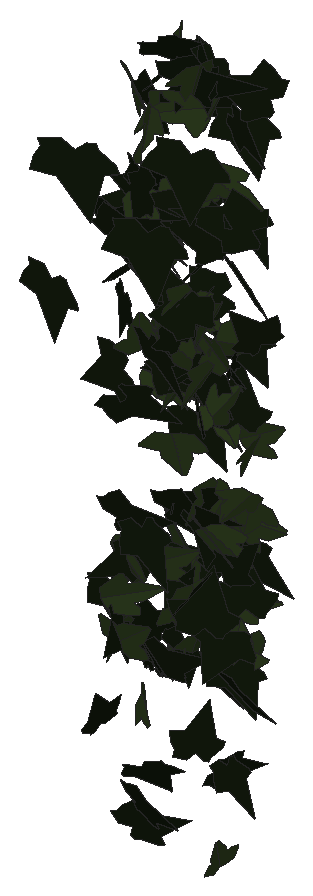
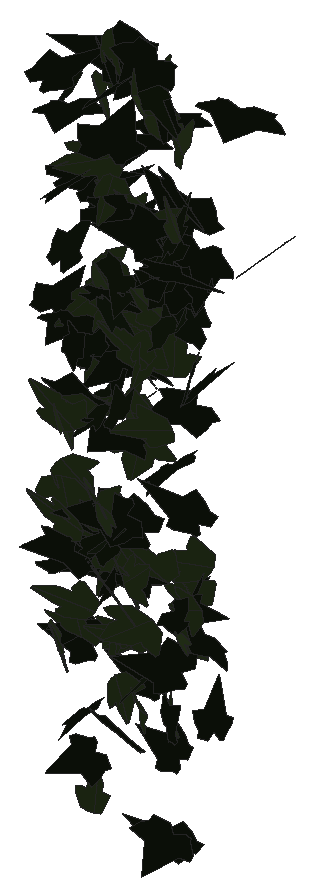
# SketchUp Ruby script. Lengths in inches.
U = 1.inch
M = Sketchup.active_model
def pt(a) = Geom::Point3d.new(a.map { |v| v * U })
def face(e, loops, mat)
  f = e.add_face(loops[0].map { |a| pt(a) })
  loops[1..].each { |l| e.add_face(l.map { |a| pt(a) }).erase! }
  f.material = f.back_material = mat if mat
  f
end
# faces: each face lists its corners as indices into pts; further lists are holes
def faces(e, pts, list, mat = nil) = list.each { |f| face(e, (f[0].is_a?(Array) ? f : [f]).map { |l| l.map { |i| pts[i] } }, mat) }
# xy, xz, yz: faces in a plane at the given z, y or x. An outline is a flat list of corners, or four numbers for a rectangle; further outlines are holes
def ring(l) = l.size == 4 ? [[l[0], l[1]], [l[2], l[1]], [l[2], l[3]], [l[0], l[3]]] : l.each_slice(2).to_a
def flat(e, list, mat, &to3) = list.each { |f| face(e, (f[0].is_a?(Array) ? f : [f]).map { |l| ring(l).map { |u, v| to3.(u, v) } }, mat) }
def xy(e, z, list, mat = nil) = flat(e, list, mat) { |x, y| [x, y, z] }
def xz(e, y, list, mat = nil) = flat(e, list, mat) { |x, z| [x, y, z] }
def yz(e, x, list, mat = nil) = flat(e, list, mat) { |y, z| [x, y, z] }
def lines(e, pts, list) = list.each { |a, b| e.add_line(pt(pts[a]), pt(pts[b])) }
# prism: a flat outline (further loops are holes) pulled along v
def prism(e, loops, v, mat = nil)
  f = face(e, loops, mat); d = Geom::Vector3d.new(v.map { |x| x * U })
  f.pushpull(f.normal.samedirection?(d) ? d.length : -d.length)
end
def box(e, o, s, mat = nil) = prism(e, [[o, [o[0] + s[0], o[1], o[2]], [o[0] + s[0], o[1] + s[1], o[2]], [o[0], o[1] + s[1], o[2]]]], [0, 0, s[2]], mat)
def at(x, y, z, deg = 0) = Geom::Transformation.translation(pt([x, y, z])) * Geom::Transformation.rotation(ORIGIN, Z_AXIS, deg.degrees)
def axes(o, x, y, z) = Geom::Transformation.new([*x, 0, *y, 0, *z, 0, *pt(o).to_a, 1])
def part(name) = M.definitions.add(name)
# library, detail: a bought-in or finely detailed component or shape, given as its bounding box
def library(name, o, s) = part(name).tap { |d| box(d.entities, o, s) }
def detail(e, o, s) = box(e.add_group.entities, o, s)
def put(e, d, t, mat = nil) = e.add_instance(d, t).tap { |i| i.material = mat if mat }
def group(e, t, mat = nil) = e.add_group.tap { |g| g.transformation = t; g.material = mat if mat }.entities
root = M.entities
M.materials.add("1026 AP 7946 SUNNY SIDE UP").color = [254, 231, 186]
M.materials.add("efeu1").color = [18, 25, 13]
M.materials.add("efeu2").color = [43, 57, 29]
c1 = part("ivyleaf_9")
p = [[1.54,2.16,1.25],[1.36,2.04,1.19],[-0.21,0.99,0.68],[-0.71,1.11,0.82],[-0.85,0.86,0.67],[-0.8,0.17,0.21],
  [-0.9,-0.01,0.1],[-0.67,-0.16,-0.02],[-0.08,-0.08,-0.05],[-0.03,-0.6,-0.4],[0.65,-0.88,-0.66],[0.83,-0.6,-0.49],
  [1.29,-0.42,-0.43],[1.8125,-0.07,-0.26],[1.21,0.44,0.15]]
faces(c1.entities,p,[[0,1,2,3,4,5,6,7,8,9,10,11,12,13,14]],"efeu1")
c2 = part("ivyleaf_10")
p = [[0,0.5,-0.03],[-0.0625,2.02,-0.43],[-0.19,2.01,-0.46],[-0.54,1.05,-0.29],[-0.52,0.625,-0.18],[-0.83,0.76,-0.28],
  [-1.16,0.64,-0.33],[-1.15,0.33,-0.24],[-0.77,-0.39,0.02],[-0.3,-0.51,0.16],[0.04,-0.48,0.23],[-0.02,2.01,-0.4375],
  [-0.06,2.01,-0.43],[0.04,-0.49,0.23],[0.67,-0.49,0.14],[1.38,0.36,-0.2],[1.375,0.51,-0.24],[0.81,0.65,-0.19],
  [0.62,0.59,-0.15],[0.6,1.09,-0.28],[0.5,1.23,-0.31]]
faces(c2.entities,p,[[0,1,2,3,4,5,6,7,8,9,10],[11,12,0,13,14,15,16,17,18,19,20]],"efeu2")
put(root,c1,axes([121.75,208.88,265.58],[-0.19201,-0.31929,-0.11255],[0.08789,0.09349,-0.35114],[0.52237,-0.1331,0.01771]),"1026 AP 7946 SUNNY SIDE UP")
put(root,c1,axes([119.59,209.1,263.89],[-0.01059,-0.33233,0.09962],[-0.00328,-0.09857,-0.34301],[0.54506,-0.00705,-0.00013]),"1026 AP 7946 SUNNY SIDE UP")
put(root,c1,axes([120.09,209.08,266.43],[-0.28859,-0.21576,-0.21786],[0.23882,0.14635,-0.29045],[0.40909,-0.23764,0.01587]),"1026 AP 7946 SUNNY SIDE UP")
put(root,c2,axes([122.375,209.58,262.97],[0.06672,-0.23881,0.21649],[0.04615,-0.20954,-0.25103],[0.49948,0.05126,-0.00572]),"1026 AP 7946 SUNNY SIDE UP")
put(root,c1,axes([121.18,209.46,259.69],[0.07711,-0.30009,-0.11327],[-0.0425,0.10522,-0.31249],[0.49982,0.05524,-0.0091]),"1026 AP 7946 SUNNY SIDE UP")
put(root,c2,axes([121.8,209.7,264.09],[0.07309,-0.17687,0.28511],[0.07156,-0.27437,-0.18944],[0.51282,0.06349,-0.0142]),"1026 AP 7946 SUNNY SIDE UP")
put(root,c2,axes([120.71,209.5,257.46],[-0.38346,-0.00104,0.19279],[0.29295,0.0277,0.25043],[-0.02781,0.30615,-0.0202]),"1026 AP 7946 SUNNY SIDE UP")
put(root,c1,axes([120.51,209.78,257.6],[0.09668,-0.13183,-0.3009],[0.32323,-0.21095,0.1418],[-0.38515,-0.21013,0.04347]),"1026 AP 7946 SUNNY SIDE UP")
put(root,c1,axes([120.93,209.65,254.5],[0.14345,-0.11071,0.24535],[0.21933,-0.19398,-0.14869],[0.35096,0.16648,-0.00736]),"1026 AP 7946 SUNNY SIDE UP")
put(root,c1,axes([122.14,209.57,263.83],[-0.33863,-0.23536,0.09905],[0.0776,0.08669,0.32844],[-0.39298,0.21993,-0.0205]),"1026 AP 7946 SUNNY SIDE UP")
put(root,c2,axes([121.04,209.87,267.11],[0.00558,0.19788,-0.2247],[-0.01281,-0.2191,-0.20515],[-0.46421,0.00843,0.00296]),"1026 AP 7946 SUNNY SIDE UP")
put(root,c2,axes([120.51,209.6,258.16],[-0.04198,-0.07347,0.31793],[0.18585,0.28555,0.08213],[-0.46359,0.12113,0.00414]),"1026 AP 7946 SUNNY SIDE UP")
put(root,c1,axes([122.29,209.69,258.23],[-0.35316,-0.0801,0.21182],[0.28082,0.10742,0.24418],[-0.20493,0.28525,-0.03044]),"1026 AP 7946 SUNNY SIDE UP")
put(root,c1,axes([119.92,209.96,255.5],[0.14089,0.14245,0.24057],[-0.21769,-0.18733,0.17195],[0.3697,-0.16459,0.00957]),"1026 AP 7946 SUNNY SIDE UP")
put(root,c1,axes([120.38,209.94,264.6],[-0.11704,-0.00873,0.32962],[0.428,-0.17465,0.0593],[0.26494,0.27828,0.04982]),"1026 AP 7946 SUNNY SIDE UP")
put(root,c1,axes([121.98,209.67,258.63],[-0.16021,0.12057,-0.30094],[-0.24705,0.2478,0.16289],[0.43229,0.1863,-0.01844]),"1026 AP 7946 SUNNY SIDE UP")
put(root,c1,axes([120.82,210.15,262.71],[0.254,-0.30351,0.06175],[0.02547,-0.06118,-0.35426],[0.48633,0.16173,-0.0137]),"1026 AP 7946 SUNNY SIDE UP")
put(root,c1,axes([122.33,210.25,257.84],[-0.30263,-0.24199,0.0239],[-0.00079,-0.03094,-0.31812],[0.38247,-0.19154,0.01825]),"1026 AP 7946 SUNNY SIDE UP")
put(root,c1,axes([120.18,210.11,259.3],[0.06873,-0.00052,0.29264],[0.36819,-0.16264,-0.03838],[0.25286,0.23696,-0.02366]),"1026 AP 7946 SUNNY SIDE UP")
put(root,c2,axes([120.21,210.25,257.23],[0.097,-0.23861,0.18667],[0.05823,-0.1789,-0.25483],[0.4688,0.07159,-0.00697]),"1026 AP 7946 SUNNY SIDE UP")
put(root,c1,axes([121.37,210.2,262.95],[0.12542,0.12506,0.28018],[-0.3452,-0.16584,0.1443],[0.31849,-0.229,0.04607]),"1026 AP 7946 SUNNY SIDE UP")
put(root,c1,axes([120.01,210.39,261.82],[-0.15223,-0.10236,0.29833],[-0.19454,-0.26557,-0.14059],[0.44298,-0.1518,0.04078]),"1026 AP 7946 SUNNY SIDE UP")
put(root,c2,axes([122.14,210.29,253.53],[-0.06992,-0.24302,-0.13134],[-0.04389,-0.12307,0.25375],[-0.42827,0.05229,-0.00456]),"1026 AP 7946 SUNNY SIDE UP")
put(root,c1,axes([121.9,210.53,264.8125],[-0.08868,0.0085,0.33922],[-0.39871,-0.21427,-0.04031],[0.33046,-0.25625,0.0424]),"1026 AP 7946 SUNNY SIDE UP")
put(root,c1,axes([120.16,210.19,261.47],[0.00675,0.01487,-0.2957],[0.13792,0.27339,0.01754],[0.43052,-0.08782,-0.00098]),"1026 AP 7946 SUNNY SIDE UP")
put(root,c1,axes([120.66,210.24,265.41],[-0.13436,-0.00951,-0.29737],[-0.45069,0.03928,0.08632],[0.05505,0.29841,-0.01906]),"1026 AP 7946 SUNNY SIDE UP")
put(root,c2,axes([121.42,210.42,267.12],[0.23545,-0.00145,-0.25882],[-0.39228,-0.03537,-0.15318],[-0.04662,0.29032,-0.01823]),"1026 AP 7946 SUNNY SIDE UP")
put(root,c2,axes([122.11,210.26,262.79],[-0.20825,0.07624,-0.26325],[-0.30836,0.16619,0.1565],[0.28509,0.23545,-0.02302]),"1026 AP 7946 SUNNY SIDE UP")
put(root,c2,axes([120.29,210.54,255.79],[0.05789,-0.0084,0.30454],[0.34788,-0.19697,-0.0353],[0.30868,0.22355,-0.01733]),"1026 AP 7946 SUNNY SIDE UP")
put(root,c2,axes([121.4,210.3,262.64],[0.08609,0.01098,0.29654],[-0.44399,0.05972,0.05334],[-0.08915,-0.2868,0.0207]),"1026 AP 7946 SUNNY SIDE UP")
put(root,c2,axes([121.81,210.5,263.49],[0.05261,-0.29748,0.11628],[0.01945,-0.1139,-0.30907],[0.50088,0.03567,-0.00022]),"1026 AP 7946 SUNNY SIDE UP")
put(root,c1,axes([122.21,210.39,255.25],[0.1171,-0.22856,-0.13159],[-0.06741,0.119,-0.24692],[0.40514,0.08586,-0.00305]),"1026 AP 7946 SUNNY SIDE UP")
put(root,c2,axes([120.63,210.63,266.82],[0.05273,-0.10794,0.30341],[0.08418,-0.29051,-0.11742],[0.4869,0.06192,-0.01256]),"1026 AP 7946 SUNNY SIDE UP")
put(root,c1,axes([121.29,210.56,266.125],[-0.27246,-0.29174,-0.10439],[0.11158,0.07353,-0.34836],[0.47175,-0.18589,0.0221]),"1026 AP 7946 SUNNY SIDE UP")
put(root,c2,axes([121.51,210.45,267.83],[-0.12212,-0.33057,0.00272],[0.00563,-0.00548,-0.34983],[0.51981,-0.0776,0.00442]),"1026 AP 7946 SUNNY SIDE UP")
put(root,c2,axes([120.28,210.58,262.33],[-0.21595,-0.27174,-0.0762],[-0.07434,-0.05714,0.3129],[-0.43591,0.14437,-0.01561]),"1026 AP 7946 SUNNY SIDE UP")
put(root,c1,axes([121.97,210.57,256.63],[0.26093,-0.13225,0.19902],[0.22403,-0.13201,-0.2191],[0.29334,0.21845,-0.0097]),"1026 AP 7946 SUNNY SIDE UP")
put(root,c1,axes([121.69,210.53,262.39],[-0.04033,-0.04075,-0.34353],[-0.46758,-0.15235,0.04188],[-0.24499,0.29747,-0.02338]),"1026 AP 7946 SUNNY SIDE UP")
put(root,c2,axes([121.5,210.4375,258.28],[-0.25157,-0.22925,-0.14714],[0.15109,0.10522,-0.28688],[0.39577,-0.18589,0.01599]),"1026 AP 7946 SUNNY SIDE UP")
put(root,c2,axes([120.31,210.46,265.05],[0.14726,0.26477,0.06536],[0.05287,0.05373,-0.28867],[-0.42428,0.09859,-0.01329]),"1026 AP 7946 SUNNY SIDE UP")
put(root,c1,axes([120.2,210.49,253.43],[0.01823,0.00687,0.27088],[0.39868,-0.07018,-0.01004],[0.10982,0.25363,-0.00852]),"1026 AP 7946 SUNNY SIDE UP")
put(root,c1,axes([121.1875,210.42,267.53],[0.1974,0.03325,0.33804],[0.51819,-0.02006,-0.12799],[0.01093,0.35058,-0.03731]),"1026 AP 7946 SUNNY SIDE UP")
put(root,c1,axes([120.35,210.67,266.71],[0.00886,0.02155,0.32359],[0.20957,-0.28464,0.016],[0.4483,0.13264,-0.01388]),"1026 AP 7946 SUNNY SIDE UP")
put(root,c1,axes([119.59,210.7,264],[0.32194,-0.10366,-0.23916],[0.36648,-0.0407,0.23083],[-0.1576,-0.30641,0.04822]),"1026 AP 7946 SUNNY SIDE UP")
put(root,c1,axes([119.6,210.62,257.64],[-0.22943,-0.04689,-0.27568],[0.4167,0.04095,-0.15617],[0.09219,-0.3018,0.0198]),"1026 AP 7946 SUNNY SIDE UP")
put(root,c2,axes([120.7,210.61,262.77],[-0.00041,-0.03982,0.31346],[0.47925,-0.03726,-0.00497],[0.05903,0.30221,0.04251]),"1026 AP 7946 SUNNY SIDE UP")
put(root,c1,axes([121.62,210.42,261.35],[0.00737,-0.13117,0.31896],[-0.00051,0.31038,0.13697],[-0.5298,-0.00212,0.00431]),"1026 AP 7946 SUNNY SIDE UP")
put(root,c1,axes([120.25,210.72,256.6],[0.07254,-0.13031,0.2315],[0.11662,-0.2129,-0.14365],[0.3925,0.08734,-0.0001]),"1026 AP 7946 SUNNY SIDE UP")
put(root,c1,axes([122.38,210.7,265.11],[-0.2384,0.01588,0.30152],[-0.4452,-0.09282,-0.1465],[0.11872,-0.3162,0.05613]),"1026 AP 7946 SUNNY SIDE UP")
put(root,c2,axes([120,210.74,257.64],[0.14191,-0.18027,0.20586],[0.13149,-0.18268,-0.20869],[0.40347,0.12294,-0.00439]),"1026 AP 7946 SUNNY SIDE UP")
put(root,c2,axes([121.99,210.36,261.8],[0.04768,0.08802,-0.28926],[0.12896,0.26907,0.09742],[0.44512,-0.08739,0.00276]),"1026 AP 7946 SUNNY SIDE UP")
put(root,c1,axes([121.17,210.68,262.34],[-0.38737,0.06214,-0.12502],[0.17489,-0.05459,-0.26097],[-0.12484,-0.2693,0.02233]),"1026 AP 7946 SUNNY SIDE UP")
put(root,c2,axes([120.6,210.5625,258.41],[-0.31335,-0.07375,0.23641],[0.31802,0.11181,0.21821],[-0.20734,0.28296,-0.02259]),"1026 AP 7946 SUNNY SIDE UP")
put(root,c1,axes([122.14,210.64,256.97],[-0.08085,-0.21772,-0.14815],[0.06665,0.13638,-0.2295],[0.40375,-0.06611,0.00822]),"1026 AP 7946 SUNNY SIDE UP")
put(root,c1,axes([119.74,210.56,264.6],[0.40305,0.10824,-0.18682],[-0.24567,-0.09613,-0.2862],[-0.22468,0.29929,-0.0222]),"1026 AP 7946 SUNNY SIDE UP")
put(root,c2,axes([120.91,210.63,260.73],[-0.41776,-0.16577,-0.04424],[0.07732,0.00027,-0.32153],[0.25753,-0.26898,0.02477]),"1026 AP 7946 SUNNY SIDE UP")
put(root,c1,axes([121.01,210.64,262.23],[0.00443,-0.21174,-0.28182],[0.13631,0.26407,-0.20902],[0.52505,-0.06677,0.05664]),"1026 AP 7946 SUNNY SIDE UP")
put(root,c1,axes([122.13,210.67,267.06],[0.26584,-0.19065,-0.15826],[-0.17641,0.10414,-0.26157],[0.341,0.2025,-0.01194]),"1026 AP 7946 SUNNY SIDE UP")
put(root,c1,axes([119.9,210.93,258.11],[-0.02639,-0.0597,-0.27711],[0.03555,-0.26853,0.05846],[-0.43126,-0.01848,0.02177]),"1026 AP 7946 SUNNY SIDE UP")
put(root,c1,axes([120.69,210.69,264.61],[-0.17993,0.18896,0.1952],[0.19158,-0.14538,0.2256],[0.37329,0.1657,-0.02169]),"1026 AP 7946 SUNNY SIDE UP")
put(root,c1,axes([121.39,210.59,255.2],[-0.36933,0.15947,0.01506],[0.03551,0.00891,0.2918],[0.24916,0.23511,-0.01926]),"1026 AP 7946 SUNNY SIDE UP")
put(root,c1,axes([120.48,210.75,256.43],[0.00821,-0.00068,0.2669],[0.37041,-0.10785,-0.00582],[0.16957,0.23562,-0.00022]),"1026 AP 7946 SUNNY SIDE UP")
put(root,c2,axes([121.95,210.5625,262.97],[-0.08226,-0.15356,-0.31445],[0.22399,0.2699,-0.16393],[0.48699,-0.15008,0.02229]),"1026 AP 7946 SUNNY SIDE UP")
put(root,c1,axes([119.65,210.68,263.32],[0.10116,0.27809,0.02464],[-0.02444,-0.01932,0.29373],[0.438,-0.06531,0.0107]),"1026 AP 7946 SUNNY SIDE UP")
put(root,c2,axes([119.61,210.88,258.21],[-0.18796,0.08873,-0.24765],[0.26808,-0.17122,-0.15313],[-0.30178,-0.20737,0.01821]),"1026 AP 7946 SUNNY SIDE UP")
put(root,c1,axes([120.99,210.94,258.38],[-0.34482,-0.18523,-0.02071],[0.0476,-0.00643,-0.29469],[0.2889,-0.22003,0.02384]),"1026 AP 7946 SUNNY SIDE UP")
put(root,c2,axes([120.76,211.02,261.625],[0.08003,-0.13274,0.2812],[0.11177,-0.26464,-0.14739],[0.46509,0.08644,-0.01297]),"1026 AP 7946 SUNNY SIDE UP")
put(root,c1,axes([120.63,210.75,267.38],[-0.17674,0.2587,-0.07],[0.02828,-0.06782,-0.29079],[-0.42022,-0.11337,0.00987]),"1026 AP 7946 SUNNY SIDE UP")
put(root,c1,axes([121.59,211,262.28],[0.06088,-0.14121,0.27775],[0.15083,-0.25312,-0.1518],[0.45534,0.10272,0.01315]),"1026 AP 7946 SUNNY SIDE UP")
put(root,c1,axes([121.78,210.78,258.57],[-0.18977,0.06493,0.23411],[0.31221,-0.10977,0.14053],[0.20053,0.23236,0.00274]),"1026 AP 7946 SUNNY SIDE UP")
put(root,c2,axes([120.72,210.84,265.0625],[0.19941,-0.09069,-0.28772],[0.43316,-0.06703,0.15117],[-0.15768,-0.29884,0.05141]),"1026 AP 7946 SUNNY SIDE UP")
put(root,c2,axes([121.58,210.79,265.75],[-0.27935,-0.06328,-0.28305],[0.43962,-0.00093,-0.18627],[0.05283,-0.32689,0.05333]),"1026 AP 7946 SUNNY SIDE UP")
put(root,c2,axes([121.61,210.8,259.16],[-0.32389,-0.03337,-0.20487],[0.31598,-0.01391,-0.21231],[0.02243,-0.28585,0.03255]),"1026 AP 7946 SUNNY SIDE UP")
put(root,c2,axes([122.13,210.93,259.97],[-0.18669,-0.18741,0.15261],[-0.10666,-0.1334,-0.22901],[0.36125,-0.13624,0.01125]),"1026 AP 7946 SUNNY SIDE UP")
put(root,c2,axes([121.57,210.87,267.14],[0.16965,-0.2806,-0.00647],[-0.01008,0.00256,-0.30964],[0.44116,0.10797,-0.00458]),"1026 AP 7946 SUNNY SIDE UP")
put(root,c1,axes([122.24,210.94,263.78],[0.19426,-0.27996,0.10242],[-0.04089,0.0988,0.31543],[-0.46619,-0.12532,0.01502]),"1026 AP 7946 SUNNY SIDE UP")
put(root,c1,axes([121.19,211.08,259.02],[-0.026,-0.24352,0.19859],[0.03288,-0.19485,-0.25109],[0.48861,0.00015,0.02746]),"1026 AP 7946 SUNNY SIDE UP")
put(root,c2,axes([121.02,210.91,258.41],[0.35487,-0.2075,0.00924],[-0.01091,-0.02251,-0.3152],[0.32648,0.22479,-0.02058]),"1026 AP 7946 SUNNY SIDE UP")
put(root,c2,axes([119.7,211.04,266.7],[-0.13594,-0.02207,0.33931],[0.41021,-0.21339,0.05454],[0.31836,0.26553,0.0746]),"1026 AP 7946 SUNNY SIDE UP")
put(root,c1,axes([120.6875,210.86,259.27],[0.1837,-0.03222,0.28981],[0.4135,-0.10101,-0.12494],[0.16583,0.28755,-0.0095]),"1026 AP 7946 SUNNY SIDE UP")
put(root,c1,axes([121.51,210.69,267.37],[0.06837,0.00137,0.29966],[-0.06852,0.29082,0.007],[-0.45221,-0.04386,0.04424]),"1026 AP 7946 SUNNY SIDE UP")
put(root,c1,axes([121.4,211.05,265.04],[-0.14292,-0.17214,-0.28002],[-0.20716,-0.23666,0.19912],[-0.46011,0.16002,-0.00267]),"1026 AP 7946 SUNNY SIDE UP")
put(root,c1,axes([120.54,210.71,267.89],[0.34735,0.18164,0.051],[0.08197,0.01267,-0.2936],[-0.28401,0.2258,-0.02237]),"1026 AP 7946 SUNNY SIDE UP")
put(root,c2,axes([121.3,210.76,263.28],[0.03746,0.26838,0.14568],[0.01649,0.13951,-0.27675],[-0.47561,0.02598,0.00188]),"1026 AP 7946 SUNNY SIDE UP")
put(root,c1,axes([122.37,211.01,262.89],[0.11073,0.07576,0.25743],[-0.34812,-0.11907,0.10094],[0.21647,-0.23024,0.03065]),"1026 AP 7946 SUNNY SIDE UP")
put(root,c1,axes([121.23,211.11,258.07],[-0.05735,-0.03883,0.28179],[-0.19224,-0.2454,-0.05408],[0.38995,-0.12669,0.01478]),"1026 AP 7946 SUNNY SIDE UP")
put(root,c1,axes([119.9,211.13,264.86],[0.24613,-0.2832,-0.12325],[0.17937,-0.06929,0.32671],[-0.44785,-0.18339,0.06311]),"1026 AP 7946 SUNNY SIDE UP")
put(root,c2,axes([120.81,210.84,257.51],[-0.18418,-0.19921,-0.13906],[0.15365,0.09645,-0.23541],[0.34468,-0.14944,0.03063]),"1026 AP 7946 SUNNY SIDE UP")
put(root,c1,axes([119.93,211.04,264.59],[0.1976,-0.18737,0.18648],[0.17634,-0.1438,-0.23302],[0.37104,0.16813,0.01144]),"1026 AP 7946 SUNNY SIDE UP")
put(root,c1,axes([122.22,210.8125,258.06],[-0.3709,-0.11251,0.1814],[0.23224,0.09942,0.26888],[-0.23361,0.27746,-0.02069]),"1026 AP 7946 SUNNY SIDE UP")
put(root,c1,axes([122.08,210.99,265.24],[0.06861,-0.28914,-0.05831],[-0.00077,0.05549,-0.30081],[0.46278,0.04296,0.00814]),"1026 AP 7946 SUNNY SIDE UP")
put(root,c2,axes([122.27,210.96,261.01],[0.09918,-0.31307,0.00053],[-0.00992,-0.00361,-0.32895],[0.49219,0.06301,-0.00674]),"1026 AP 7946 SUNNY SIDE UP")
put(root,c2,axes([121.97,210.87,256.99],[0.4739,-0.03798,0.02041],[-0.02367,0.03953,0.31081],[-0.06322,-0.29945,0.03663]),"1026 AP 7946 SUNNY SIDE UP")
put(root,c1,axes([119.92,211.13,263.28],[0.0884,-0.26216,0.17147],[0.07052,-0.16205,-0.27703],[0.48444,0.07143,0.00904]),"1026 AP 7946 SUNNY SIDE UP")
put(root,c1,axes([120.05,211.1,264],[0.16311,-0.18337,0.20291],[0.11702,-0.18447,-0.21724],[0.4079,0.12625,-0.01882]),"1026 AP 7946 SUNNY SIDE UP")
put(root,c1,axes([121.43,211.07,258.71],[0.28615,-0.24512,0.06513],[-0.03656,0.06306,0.3143],[-0.39692,-0.18253,0.018]),"1026 AP 7946 SUNNY SIDE UP")
put(root,c1,axes([121.93,211.12,262.55],[-0.15706,0.06799,-0.27495],[0.26555,-0.20966,-0.12118],[-0.34284,-0.19354,0.03209]),"1026 AP 7946 SUNNY SIDE UP")
put(root,c2,axes([121.55,210.92,261.36],[0.27949,0.18589,0.1017],[0.12917,0.0562,-0.26389],[-0.30386,0.19487,-0.01863]),"1026 AP 7946 SUNNY SIDE UP")
put(root,c1,axes([121.48,211.07,263.43],[-0.37074,0.00045,0.1471],[-0.22363,-0.02518,-0.24201],[0.01991,-0.27449,0.02082]),"1026 AP 7946 SUNNY SIDE UP")
put(root,c1,axes([119.42,211.19,262.625],[0.09102,-0.07609,-0.29034],[0.35432,-0.17033,0.0942],[-0.29079,-0.23136,0.0239]),"1026 AP 7946 SUNNY SIDE UP")
put(root,c1,axes([119.97,210.81,256.91],[0.11279,0.04282,0.30319],[0.42929,0.10994,-0.08446],[-0.18448,0.28201,-0.01117]),"1026 AP 7946 SUNNY SIDE UP")
put(root,c2,axes([121.18,211.19,259.67],[0.07546,-0.22563,0.22805],[0.05333,-0.22024,-0.23875],[0.49558,0.05806,-0.00903]),"1026 AP 7946 SUNNY SIDE UP")
put(root,c1,axes([121.03,211.05,261.06],[-0.17676,-0.12302,-0.24354],[0.30103,0.14012,-0.16859],[0.2901,-0.22036,0.02655]),"1026 AP 7946 SUNNY SIDE UP")
put(root,c2,axes([120.53,211.05,261.53],[0.02057,-0.00691,0.29569],[0.44989,0.0246,-0.01268],[-0.03816,0.28631,0.00991]),"1026 AP 7946 SUNNY SIDE UP")
put(root,c2,axes([121.53,211.08,259.76],[0.29743,-0.24642,-0.01036],[-0.02905,-0.00328,-0.31959],[0.38663,0.18933,-0.01604]),"1026 AP 7946 SUNNY SIDE UP")
put(root,c1,axes([121.9375,211.04,262.82],[-0.10777,-0.17984,-0.194],[0.12974,0.16859,-0.19688],[0.38713,-0.10657,0.01197]),"1026 AP 7946 SUNNY SIDE UP")
put(root,c2,axes([121.23,210.9375,265.45],[-0.11171,-0.25964,-0.17231],[0.09545,0.155,-0.27598],[0.47489,-0.09223,0.01493]),"1026 AP 7946 SUNNY SIDE UP")
put(root,c1,axes([121.11,210.81,263.79],[0.04439,0.24631,0.17799],[0.03423,0.16999,-0.2544],[-0.47057,0.0356,-0.00172]),"1026 AP 7946 SUNNY SIDE UP")
put(root,c1,axes([121.31,211.04,261.45],[0.32225,-0.18709,-0.09096],[-0.12421,0.04249,-0.28482],[0.29989,0.21865,-0.02022]),"1026 AP 7946 SUNNY SIDE UP")
put(root,c1,axes([121.22,211.125,263.42],[-0.26264,0.15036,-0.16147],[0.14867,-0.12886,-0.23065],[-0.30855,-0.19008,0.02631]),"1026 AP 7946 SUNNY SIDE UP")
put(root,c1,axes([121.96,211.14,266.78],[-0.14281,-0.2646,-0.1291],[0.06699,0.11628,-0.28751],[0.45444,-0.10029,0.00181]),"1026 AP 7946 SUNNY SIDE UP")
put(root,c1,axes([119.68,211.09,264.18],[0.38005,-0.11635,0.10842],[0.13117,-0.06981,-0.27556],[0.20975,0.25448,-0.02411]),"1026 AP 7946 SUNNY SIDE UP")
put(root,c1,axes([121.94,210.96,261.33],[-0.44329,0.06215,0.08593],[0.13389,0.00129,0.29678],[0.09316,0.29389,-0.01768]),"1026 AP 7946 SUNNY SIDE UP")
put(root,c1,axes([121.6875,210.85,254.84],[-0.01333,0.11713,-0.2649],[-0.08688,0.25228,0.12143],[0.43669,0.05376,0.01607]),"1026 AP 7946 SUNNY SIDE UP")
put(root,c1,axes([122.28,211.3,267.22],[-0.06264,0.00941,0.34615],[-0.43816,-0.19006,-0.02967],[0.29544,-0.27987,0.02939]),"1026 AP 7946 SUNNY SIDE UP")
put(root,c2,axes([120.43,211,262.74],[-0.09519,-0.25173,-0.18694],[0.10844,0.16786,-0.2647],[0.47439,-0.08888,0.023]),"1026 AP 7946 SUNNY SIDE UP")
put(root,c2,axes([122.11,211.12,259.72],[-0.42867,-0.0474,0.06886],[-0.09375,-0.0459,-0.28317],[0.0889,-0.27698,0.03343]),"1026 AP 7946 SUNNY SIDE UP")
put(root,c2,axes([122.03,211.1,260.97],[-0.35158,-0.01144,0.23361],[0.34903,0.05635,0.22867],[-0.07557,0.31348,-0.03068]),"1026 AP 7946 SUNNY SIDE UP")
put(root,c2,axes([120.32,211.03,263.52],[0.10765,-0.24486,0.14075],[-0.00035,0.142,0.26049],[-0.44197,-0.05975,0.03408]),"1026 AP 7946 SUNNY SIDE UP")
put(root,c1,axes([120.99,210.93,259.5],[0.10669,0.13543,-0.26855],[0.14585,0.24481,0.15687],[0.43941,-0.11414,0.01314]),"1026 AP 7946 SUNNY SIDE UP")
put(root,c1,axes([120.21,211.16,264.9375],[0.31713,-0.09187,0.1991],[0.2518,-0.11244,-0.22726],[0.22431,0.2561,-0.02638]),"1026 AP 7946 SUNNY SIDE UP")
put(root,c2,axes([120.75,211.13,257.48],[0.33286,0.06507,0.17169],[0.25736,0.03242,-0.22753],[-0.11227,0.26723,-0.01252]),"1026 AP 7946 SUNNY SIDE UP")
put(root,c2,axes([120.83,210.96,257.36],[0.12516,0.03616,-0.30101],[0.34576,0.19428,0.08756],[0.30831,-0.23256,0.024]),"1026 AP 7946 SUNNY SIDE UP")
put(root,c2,axes([120.47,211.18,262.71],[-0.21479,0.00909,0.29355],[0.44744,0.02271,0.13994],[-0.02605,0.31513,-0.0167]),"1026 AP 7946 SUNNY SIDE UP")
put(root,c1,axes([120.52,211.36,256.58],[0.01206,-0.25271,0.11835],[0.01355,-0.11609,-0.2611],[0.43723,0.01057,0.00482]),"1026 AP 7946 SUNNY SIDE UP")
put(root,c2,axes([120.71,211.1,258.46],[-0.27161,0.16476,-0.20068],[-0.19817,0.15072,0.24617],[0.3501,0.21314,-0.01634]),"1026 AP 7946 SUNNY SIDE UP")
put(root,c2,axes([120.12,211.11,261.45],[0.10434,0.04675,0.28963],[0.33204,0.18539,-0.0821],[-0.30035,0.22119,0.00986]),"1026 AP 7946 SUNNY SIDE UP")
put(root,c1,axes([121.02,211.47,267.43],[-0.11077,-0.24931,0.14209],[-0.04603,-0.13646,-0.26757],[0.44673,-0.07588,0.00766]),"1026 AP 7946 SUNNY SIDE UP")
put(root,c1,axes([121.77,211.28,258.72],[0.01995,-0.08747,-0.29056],[0.40951,0.13541,-0.03046],[0.21728,-0.24718,0.08408]),"1026 AP 7946 SUNNY SIDE UP")
put(root,c1,axes([120.04,211.35,264.53],[-0.36444,0.02509,0.16798],[-0.25907,-0.02643,-0.23743],[-0.00814,-0.28207,0.03551]),"1026 AP 7946 SUNNY SIDE UP")
put(root,c1,axes([121.28,211.05,258.18],[-0.11471,0.21357,0.25852],[-0.16223,0.22799,-0.23058],[-0.49057,-0.12533,0.0158]),"1026 AP 7946 SUNNY SIDE UP")
put(root,c1,axes([119.9,211.17,256.11],[0.06667,-0.11037,0.25296],[-0.03923,0.24652,0.11974],[-0.42239,-0.04032,0.02881]),"1026 AP 7946 SUNNY SIDE UP")
put(root,c2,axes([119.63,211.32,265.34],[0.13685,-0.25001,-0.05513],[0.04054,-0.04616,0.27229],[-0.39951,-0.09032,0.00874]),"1026 AP 7946 SUNNY SIDE UP")
put(root,c2,axes([121.75,211.37,259.25],[0.08448,-0.07467,-0.33572],[0.45037,-0.15914,0.08539],[-0.26988,-0.28894,0.03741]),"1026 AP 7946 SUNNY SIDE UP")
put(root,c2,axes([120.5,211.15,256.16],[0.18664,-0.07211,0.24478],[-0.29053,0.15097,0.14293],[-0.26176,-0.21898,0.01589]),"1026 AP 7946 SUNNY SIDE UP")
put(root,c1,axes([119.85,211.15,254.1],[0.3143,0.17283,0.00658],[0.02174,-0.00774,-0.27184],[-0.27103,0.19981,-0.01418]),"1026 AP 7946 SUNNY SIDE UP")
put(root,c2,axes([120.32,211.46,267.66],[0.15478,-0.09609,0.25645],[0.24214,-0.19694,-0.14189],[0.34363,0.18206,-0.01553]),"1026 AP 7946 SUNNY SIDE UP")
put(root,c2,axes([122.12,211.28,257.08],[0.20428,-0.24519,-0.0663],[-0.05318,0.05332,-0.2855],[0.39447,0.13416,-0.00416]),"1026 AP 7946 SUNNY SIDE UP")
put(root,c2,axes([121.61,211.23,257.73],[-0.13918,-0.03108,0.28563],[0.34802,0.16956,0.09331],[-0.26752,0.23675,-0.02721]),"1026 AP 7946 SUNNY SIDE UP")
put(root,c1,axes([120.36,211.5,261.93],[0.00938,-0.30052,0.06358],[0.00606,-0.06336,-0.31001],[0.4829,0.00663,0.00265]),"1026 AP 7946 SUNNY SIDE UP")
put(root,c1,axes([120.89,211.4375,266.4375],[0.2548,0.09633,0.26834],[-0.38411,-0.0927,0.19173],[0.20603,-0.29194,0.0256]),"1026 AP 7946 SUNNY SIDE UP")
put(root,c1,axes([120.61,211.55,261.7],[-0.004,-0.14853,0.24226],[0.03613,-0.23532,-0.1537],[0.43698,0.0181,0.01493]),"1026 AP 7946 SUNNY SIDE UP")
put(root,c2,axes([120.72,211.38,256.65],[-0.06591,-0.29269,0.00649],[0.00594,-0.00859,-0.30462],[0.46037,-0.04179,0.00486]),"1026 AP 7946 SUNNY SIDE UP")
put(root,c2,axes([120.32,211.35,257.91],[-0.39612,0.00243,-0.22123],[0.33455,-0.04235,-0.25786],[-0.04608,-0.32832,0.02967]),"1026 AP 7946 SUNNY SIDE UP")
